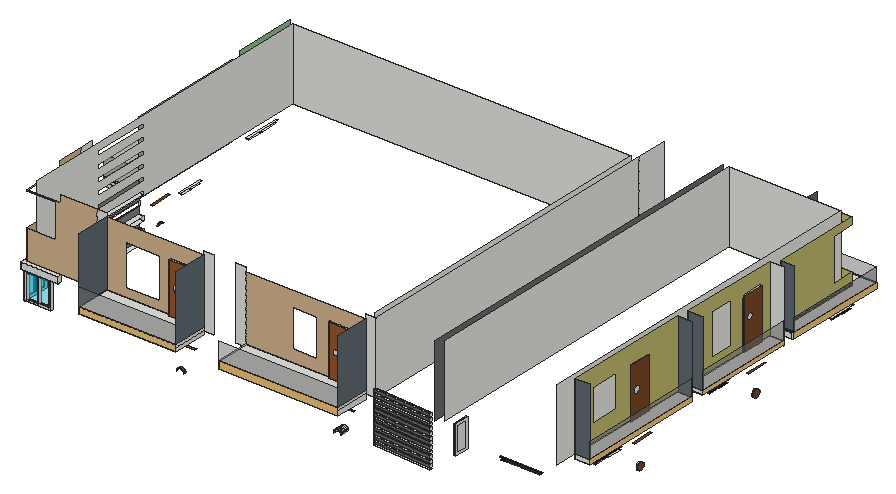
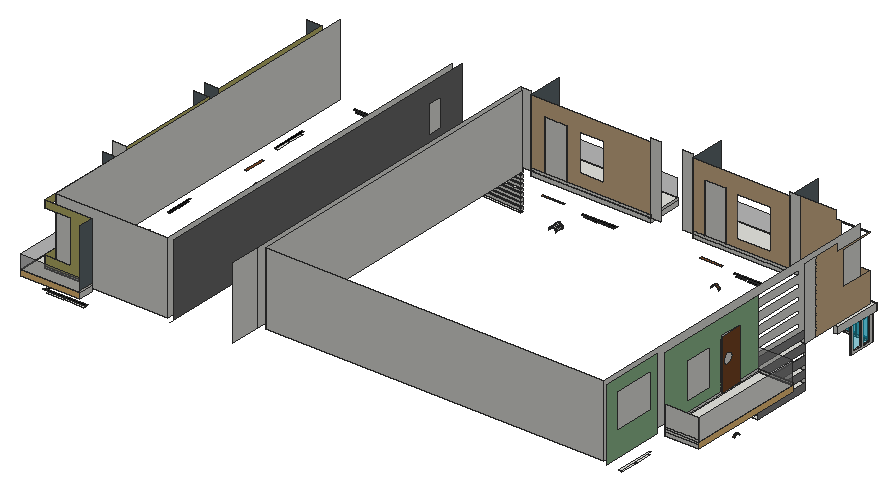
# SketchUp Ruby script. Lengths in inches.
U = 1.inch
M = Sketchup.active_model
def pt(a) = Geom::Point3d.new(a.map { |v| v * U })
def face(e, loops, mat)
  f = e.add_face(loops[0].map { |a| pt(a) })
  loops[1..].each { |l| e.add_face(l.map { |a| pt(a) }).erase! }
  f.material = f.back_material = mat if mat
  f
end
# faces: each face lists its corners as indices into pts; further lists are holes
def faces(e, pts, list, mat = nil) = list.each { |f| face(e, (f[0].is_a?(Array) ? f : [f]).map { |l| l.map { |i| pts[i] } }, mat) }
# xy, xz, yz: faces in a plane at the given z, y or x. An outline is a flat list of corners, or four numbers for a rectangle; further outlines are holes
def ring(l) = l.size == 4 ? [[l[0], l[1]], [l[2], l[1]], [l[2], l[3]], [l[0], l[3]]] : l.each_slice(2).to_a
def flat(e, list, mat, &to3) = list.each { |f| face(e, (f[0].is_a?(Array) ? f : [f]).map { |l| ring(l).map { |u, v| to3.(u, v) } }, mat) }
def xy(e, z, list, mat = nil) = flat(e, list, mat) { |x, y| [x, y, z] }
def xz(e, y, list, mat = nil) = flat(e, list, mat) { |x, z| [x, y, z] }
def yz(e, x, list, mat = nil) = flat(e, list, mat) { |y, z| [x, y, z] }
def lines(e, pts, list) = list.each { |a, b| e.add_line(pt(pts[a]), pt(pts[b])) }
# prism: a flat outline (further loops are holes) pulled along v
def prism(e, loops, v, mat = nil)
  f = face(e, loops, mat); d = Geom::Vector3d.new(v.map { |x| x * U })
  f.pushpull(f.normal.samedirection?(d) ? d.length : -d.length)
end
def box(e, o, s, mat = nil) = prism(e, [[o, [o[0] + s[0], o[1], o[2]], [o[0] + s[0], o[1] + s[1], o[2]], [o[0], o[1] + s[1], o[2]]]], [0, 0, s[2]], mat)
def at(x, y, z, deg = 0) = Geom::Transformation.translation(pt([x, y, z])) * Geom::Transformation.rotation(ORIGIN, Z_AXIS, deg.degrees)
def axes(o, x, y, z) = Geom::Transformation.new([*x, 0, *y, 0, *z, 0, *pt(o).to_a, 1])
def part(name) = M.definitions.add(name)
# library, detail: a bought-in or finely detailed component or shape, given as its bounding box
def library(name, o, s) = part(name).tap { |d| box(d.entities, o, s) }
def detail(e, o, s) = box(e.add_group.entities, o, s)
def put(e, d, t, mat = nil) = e.add_instance(d, t).tap { |i| i.material = mat if mat }
def group(e, t, mat = nil) = e.add_group.tap { |g| g.transformation = t; g.material = mat if mat }.entities
root = M.entities
M.materials.add("[0035_Tan]").color = [210, 180, 140]
M.materials.add("[0057_DarkKhaki]").color = [189, 183, 107]
M.materials.add("[0072_DarkSeaGreen]").color = [143, 188, 143]
M.materials.add("[0133_Gray]").color = [128, 128, 128]
M.materials.add("[0134_DimGray]").color = [105, 105, 105]
M.materials.add("[0137_Black]").color = [0, 0, 0]
M.materials.add("[Formica Speckled Grey]").color = [94, 105, 111]
M.materials.add("[Translucent Glass Gray]").color = [128, 128, 128]
M.materials["[Translucent Glass Gray]"].alpha = 0.5
M.materials.add("[Translucent Glass Tinted]").color = [8, 201, 241]
M.materials["[Translucent Glass Tinted]"].alpha = 0.48
M.materials.add("[Wood Cherry Original]").color = [152, 86, 42]
M.materials.add("[Wood OSB]").color = [240, 195, 122]
M.materials.add("[Wood Veneer 01]").color = [120, 70, 37]
xy(root,300.63,[[83.8125,295.24,92.8125,392.06]])
xy(root,300.91,[[763.41,201.89,766.41,227.45]])
xy(root,303.43,[[766.19,148.96,766.41,152.52,668.06,158.52,667.84,154.96]])
xy(root,303.91,[[763.41,204.89,766.41,224.45]])
xy(root,306.11,[[766.19,148.96,667.84,154.96,668.05,158.39,766.4,152.39],[766.4,152.39,668.05,158.39,668.06,158.52,766.41,152.52]])
xy(root,310.31,[[766.19,148.96,766.4,152.39,668.05,158.39,667.84,154.96],[766.4,152.39,766.41,152.52,668.06,158.52,668.05,158.39]])
xy(root,312.98,[[766.19,148.96,667.84,154.96,668.06,158.52,766.41,152.52]])
xy(root,313.12,[[83.8125,295.24,92.8125,392.06]])
xy(root,314.18,[[83.8125,155.58,126.6875,158.58]])
xy(root,314.24,[[80.8125,155.58,83.8125,155.71],[80.8125,155.71,83.8125,200.33]])
xy(root,317.18,[[766.19,148.96,766.41,152.52,668.06,158.52,667.84,154.96],[86.8125,155.58,105.25,158.58],[106.83,155.58,123.6875,158.58]])
xy(root,317.24,[[80.8125,161.58,83.8125,177.8],[80.8125,179.46,83.8125,197.33]])
xy(root,319.86,[[766.19,148.96,667.84,154.96,668.06,158.52,766.41,152.52]])
xy(root,320.56,[[83.8125,295.24,92.8125,392.06]])
xy(root,324.06,[[766.19,148.96,766.41,152.52,668.06,158.52,667.84,154.96]])
xy(root,326.73,[[766.19,148.96,667.84,154.96,668.06,158.52,766.41,152.52]])
xy(root,329.54,[[80.8125,483.71,83.8125,500.7],[80.8125,502.52,83.8125,521.33]])
xy(root,330.93,[[766.19,148.96,766.41,152.52,668.06,158.52,667.84,154.96]])
xy(root,332.54,[[80.8125,480.71,83.8125,524.33]])
xy(root,333.06,[[83.8125,295.24,92.8125,392.06]])
xy(root,333.34,[[267.42,155.58,288.08,158.58],[291.62,155.58,308.74,158.58]],"[0137_Black]")
xy(root,333.43,[[511.66,155.58,537.16,158.58],[540.07,155.58,562.66,158.58]],"[0137_Black]")
xy(root,333.61,[[766.19,148.96,667.84,154.96,668.06,158.52,766.41,152.52]])
xy(root,336.34,[[264.42,155.58,311.74,158.58]],"[0137_Black]")
xy(root,336.43,[[508.66,155.58,565.66,158.58]],"[0137_Black]")
xy(root,337.81,[[766.19,148.96,766.41,152.52,668.06,158.52,667.84,154.96]])
xy(root,340.06,[[80.8125,421.71,83.8125,457.71]],"[Wood Veneer 01]")
xy(root,340.47,[[332.04,155.58,368.04,158.58]],"[Wood Cherry Original]")
xy(root,340.48,[[766.19,148.96,667.84,154.96,668.06,158.52,766.41,152.52]])
xy(root,340.5,[[83.8125,295.24,92.8125,392.06]])
xy(root,340.72,[[596.81,155.58,632.81,158.58]],"[Wood Cherry Original]")
xy(root,343.18,[[972.47,553.32,975.47,589.32]],"[Wood Veneer 01]")
xy(root,343.44,[[972.47,315.42,975.47,351.42]],"[Wood Veneer 01]")
xy(root,344.68,[[766.19,148.96,766.41,152.52,668.06,158.52,667.84,154.96]])
xy(root,345.53,[[763.41,204.89,766.41,224.45]])
xy(root,346.83,[[972.47,234.45,975.47,260.01],[972.47,262.22,975.47,285.58]])
xy(root,347.28,[[906.22,770.48,937.84,773.48],[940.13,770.48,969.47,773.48]])
xy(root,347.28,[[972.47,728.48,975.47,747.98],[972.47,750.32,975.47,767.48]],"[0137_Black]")
xy(root,347.36,[[766.19,148.96,667.84,154.96,668.06,158.52,766.41,152.52]])
xy(root,348.53,[[763.41,201.89,766.41,227.45]])
xy(root,349.41,[[972.47,471.54,975.47,490.38],[972.47,492.52,975.47,509.23]],"[0137_Black]")
xy(root,349.83,[[972.47,231.45,975.47,288.58]],"[0137_Black]")
xy(root,350.04,[[80.8125,623.08,83.8125,648.35],[80.8125,651.58,83.8125,680.08]])
xy(root,350.28,[[972.47,725.48,975.47,770.48]])
xy(root,350.28,[[903.22,770.48,972.47,773.48],[972.47,770.48,975.47,773.48]],"[0137_Black]")
xy(root,351.56,[[766.19,148.96,766.41,152.52,668.06,158.52,667.84,154.96]])
xy(root,352.41,[[972.47,468.54,975.47,512.23]],"[0137_Black]")
xy(root,353,[[83.8125,295.24,85.75,392.06]])
xy(root,353.04,[[80.8125,620.08,83.8125,683.08]])
xy(root,354.23,[[766.19,148.96,667.84,154.96,668.06,158.52,766.41,152.52]])
xy(root,355.59,[[914.48,155.58,916.69,158.58]])
xy(root,355.59,[[880.02,155.58,912.27,158.58],[912.27,155.58,914.48,158.58],[916.69,155.58,944.52,158.58]],"[0137_Black]")
xy(root,357.74,[[86.8125,155.58,105.25,158.58],[106.83,155.58,123.6875,158.58],[80.8125,161.58,83.8125,177.8],[80.8125,179.46,83.8125,197.33]])
xy(root,358.43,[[766.19,148.96,766.41,152.52,668.06,158.52,667.84,154.96]])
xy(root,358.59,[[877.02,155.58,947.52,158.58]],"[0137_Black]")
xy(root,360.44,[[83.8125,295.24,85.75,392.06]])
xy(root,360.74,[[77.8125,152.58,77.8125,232.98,83.8125,232.98,83.8125,200.33,80.8125,200.33,80.8125,155.58,126.6875,155.58,126.6875,158.58,141.375,158.58,141.375,152.58],[80.8125,155.58,83.8125,155.71],[83.8125,155.58,126.6875,158.58],[80.8125,155.71,83.8125,200.33]])
xy(root,361.48,[[766.19,148.96,667.84,154.96,668.06,158.52,766.41,152.52]])
xy(root,362.62,[[26.03,392.06,83.8125,587.65]],"[Wood OSB]")
xy(root,364.37,[[450.92,100.8,651.23,158.58]],"[Wood OSB]")
xy(root,365.68,[[766.19,148.96,766.41,152.52,668.06,158.52,667.84,154.96]])
xy(root,366.18,[[217.79,100.8,379.72,158.58]],"[Wood OSB]")
xy(root,368.73,[[766.19,148.96,667.84,154.96,668.06,158.52,766.41,152.52]])
xy(root,372.18,[[77.8125,152.58,141.375,152.58,141.375,158.58,83.8125,158.58,83.8125,232.98,77.8125,232.98],[26.03,392.06,83.8125,587.65]])
xy(root,372.18,[[972.47,194.93,996.47,408.53]],"[Wood OSB]")
xy(root,372.33,[[975.47,621.6875,975.47,770.48,896.3125,770.48,896.3125,794.48,996.47,794.48,996.47,621.6875]],"[Wood OSB]")
xy(root,372.5,[[972.47,431.23,996.47,600.85]],"[Wood OSB]")
xy(root,372.93,[[766.19,148.96,766.41,152.52,668.06,158.52,667.84,154.96],[83.8125,295.24,92.8125,392.06]])
xy(root,375.98,[[766.19,148.96,667.84,154.96,668.06,158.52,766.41,152.52]])
xy(root,376.06,[[80.8125,433.46,83.8125,469.46]])
xy(root,376.47,[[217.79,100.8,379.72,100.8,379.72,158.58,360.41,158.58,360.41,155.58,324.41,155.58,324.41,158.58,217.79,158.58],[324.41,155.58,360.41,158.58]])
xy(root,376.6,[[450.92,100.8,651.23,100.8,651.23,158.58,627.01,158.58,627.01,155.58,591.01,155.58,591.01,158.58,450.92,158.58],[591.01,155.58,627.01,158.58]])
xy(root,378.87,[[972.47,431.23,996.47,431.23,996.47,600.85,972.47,600.85,972.47,581.86,975.47,581.86,975.47,545.86,972.47,545.86],[972.47,545.86,975.47,581.86]])
xy(root,379.19,[[972.47,194.93,996.47,194.93,996.47,408.53,972.47,408.53,972.47,344.12,975.47,344.12,975.47,308.12,972.47,308.12],[972.47,308.12,975.47,344.12]])
xy(root,380.18,[[766.19,148.96,766.41,152.52,668.06,158.52,667.84,154.96]])
xy(root,380.38,[[83.8125,295.24,92.8125,392.06]])
xy(root,381.33,[[975.47,621.6875,996.47,621.6875,996.47,794.48,896.3125,794.48,896.3125,770.48,975.47,770.48]])
xy(root,383.23,[[766.19,148.96,667.84,154.96,668.06,158.52,766.41,152.52]])
xy(root,387.43,[[766.19,148.96,766.41,152.52,668.06,158.52,667.84,154.96]])
xz(root,100.8,[[217.79,376.47,379.72,406.08],[450.92,376.6,651.23,406.95]],"[Translucent Glass Gray]")
xz(root,100.8,[[450.92,364.37,651.23,376.6],[217.79,366.18,379.72,376.47]],"[Wood OSB]")
xz(root,152.58,[[77.8125,360.74,141.375,372.18]])
xz(root,155.58,[[[83.8125,314.18,126.6875,314.18,126.6875,360.74,80.8125,360.74,80.8125,314.24,83.8125,314.24],[86.8125,317.18,105.25,357.74],[106.83,317.18,123.6875,357.74]]])
xz(root,155.58,[[[324.41,376.47,360.41,460.47],[337.43,413.47,335.75,413.69,334.18,414.34,332.84,415.375,331.8,416.72,331.15,418.29,330.93,419.97,331.15,421.65,331.8,423.22,332.84,424.57,334.18,425.6,335.75,426.25,337.43,426.47,339.12,426.25,340.68,425.6,342.03,424.57,343.0625,423.22,343.71,421.65,343.93,419.97,343.71,418.29,343.0625,416.72,342.03,415.375,340.68,414.34,339.12,413.69]],[[591.01,376.6,627.01,460.6],[603.27,413.39,601.96,413.5625,600.74,414.07,599.69,414.87,598.89,415.92,598.38,417.14,598.21,418.45,598.38,419.76,598.89,420.98,599.69,422.03,600.74,422.83,601.96,423.34,603.27,423.51,604.58,423.34,605.81,422.83,606.85,422.03,607.66,420.98,608.16,419.76,608.34,418.45,608.16,417.14,607.66,415.92,606.85,414.87,605.81,414.07,604.58,413.5625]]],"[Wood Cherry Original]")
xz(root,158.58,[[[83.8125,314.18,126.6875,360.74],[86.8125,317.18,105.25,357.74],[106.83,317.18,123.6875,357.74]],[450.92,364.37,651.23,372.18],[217.79,366.18,379.72,372.18],[200.97,372.18,217.79,492.18],[217.79,372.18,379.72,376.47],
  [379.72,372.18,396.54,492.18],[434.03,372.18,450.85,492.18],[450.92,372.18,651.23,372.31],[651.23,372.18,668.06,492.18],[765.79,372.18,766.41,492.18],
  [450.92,372.31,651.23,376.6],[324.41,376.47,360.41,460.47],[591.01,376.6,627.01,460.6]])
xz(root,158.58,[[83.8125,372.18,200.97,372.18,200.97,492.18,140.48,492.18,140.48,479.56,83.8125,479.56,83.8125,477.85,132.6875,477.85,132.6875,421.66,83.8125,421.66],[[450.85,372.18,450.92,372.18,450.92,376.6,591.01,376.6,591.01,460.6,627.01,460.6,627.01,376.6,651.23,376.6,651.23,485.43,450.92,485.43,450.92,492.18,450.85,492.18],[528.12,396.63,569.87,459.19]],[[217.79,376.47,324.41,376.47,324.41,460.47,360.41,460.47,360.41,376.47,379.72,376.47,379.72,486.18,217.79,486.18],[249.03,390.84,306.03,458.71]]],"[0035_Tan]")
xz(root,158.58,[[86.8125,317.18,105.25,357.74],[106.83,317.18,123.6875,357.74]],"[Translucent Glass Tinted]")
xz(root,161.58,[[80.8125,317.24,83.8125,357.74]])
xz(root,177.8,[[80.8125,317.24,83.8125,357.74]])
xz(root,179.46,[[80.8125,317.24,83.8125,357.74]])
xz(root,194.93,[[972.47,372.18,996.47,379.19]])
xz(root,194.93,[[972.47,379.19,996.47,492.18]],"[Formica Speckled Grey]")
xz(root,197.33,[[80.8125,317.24,83.8125,357.74]])
xz(root,200.33,[[80.8125,314.24,83.8125,360.74]])
xz(root,201.89,[[763.41,300.91,766.41,348.53]])
xz(root,204.89,[[763.41,303.91,766.41,345.53]])
xz(root,224.45,[[763.41,303.91,766.41,345.53]])
xz(root,227.45,[[763.41,300.91,766.41,348.53]])
xz(root,232.98,[[77.8125,360.74,83.8125,372.18]])
xz(root,295.24,[[83.8125,313.12,92.8125,320.56],[83.8125,333.06,92.8125,340.5],[83.8125,353,85.75,360.44],[83.8125,372.93,92.8125,380.38]])
xz(root,308.12,[[972.47,379.19,975.47,463.19]],"[Wood Veneer 01]")
xz(root,344.12,[[972.47,379.19,975.47,463.19]],"[Wood Veneer 01]")
xz(root,392.06,[[83.8125,313.12,92.8125,320.56],[83.8125,333.06,92.8125,340.5],[83.8125,353,85.75,360.44],[26.03,362.62,83.8125,368.62],[26.03,368.62,83.8125,372.18],
  [26.03,372.18,83.8125,372.56],[26.03,372.56,83.8125,372.93],[26.03,372.93,83.8125,376.06],[83.8125,372.93,92.8125,380.38]])
xz(root,392.06,[[26.03,376.06,83.8125,409.83]],"[Translucent Glass Gray]")
xz(root,408.53,[[972.47,372.18,996.47,379.19]])
xz(root,408.53,[[972.47,379.19,996.47,492.18]],"[Formica Speckled Grey]")
xz(root,431.23,[[972.47,372.18,996.47,372.5],[972.47,372.5,996.47,378.87]])
xz(root,431.23,[[972.47,378.87,996.47,489.56]],"[Formica Speckled Grey]")
xz(root,433.46,[[80.8125,376.06,83.8125,460.06]],"[Wood Veneer 01]")
xz(root,469.46,[[80.8125,376.06,83.8125,460.06]],"[Wood Veneer 01]")
xz(root,545.86,[[972.47,378.87,975.47,462.87]],"[Wood Veneer 01]")
xz(root,581.86,[[972.47,378.87,975.47,462.87]],"[Wood Veneer 01]")
xz(root,587.65,[[26.03,362.62,83.8125,368.62],[26.03,368.62,83.8125,372.18],[26.03,372.18,83.8125,376.06],[26.03,376.06,83.8125,409.42]])
xz(root,600.85,[[972.47,372.18,996.47,372.5],[972.47,372.5,996.47,378.87],[972.47,378.87,996.47,489.56]])
xz(root,621.6875,[[975.47,372.33,993.47,381.33],[993.47,372.33,996.47,381.33],[975.47,381.33,993.47,381.52],[993.47,381.33,996.47,381.52],[975.47,381.52,993.47,383.71],
  [993.47,381.52,996.47,383.71],[975.47,383.71,993.47,384.33],[993.47,383.71,996.47,384.33]])
xz(root,621.6875,[[975.47,384.33,996.47,482.83]],"[Formica Speckled Grey]")
xz(root,703.7,[[92.8125,372.18,659.06,492.18]])
xz(root,761.48,[[775.41,372.18,963.47,492.18]])
xz(root,770.48,[[896.3125,372.33,918.4,381.33],[918.4,372.33,975.47,381.33],[896.3125,381.33,918.4,384.33],[918.4,381.33,975.47,384.33]])
xz(root,770.48,[[896.3125,384.33,896.3125,482.83,975.47,482.83,975.47,471.13,931.65,471.13,931.65,400.19,975.47,400.19,975.47,384.33]],"[0057_DarkKhaki]")
xz(root,794.48,[[896.3125,381.33,996.47,405.05]],"[Translucent Glass Gray]")
xz(root,794.48,[[896.3125,372.33,996.47,381.33]],"[Wood OSB]")
yz(root,26.03,[[392.06,372.18,587.65,409.42]],"[Translucent Glass Gray]")
yz(root,26.03,[[392.06,362.62,587.65,372.18]],"[Wood OSB]")
yz(root,77.8125,[[152.58,360.74,232.98,372.18]])
yz(root,80.8125,[[155.58,314.24,155.71,360.74],[[155.71,314.24,200.33,360.74],[179.46,317.24,197.33,357.74],[161.58,317.24,177.8,357.74]]])
yz(root,80.8125,[[[433.46,376.06,469.46,460.06],[458.74,414.24,461.07,414.54,463.24,415.44,465.1,416.87,466.53,418.74,467.43,420.91,467.74,423.24,467.43,425.57,466.53,427.74,465.1,429.6,463.24,431.03,461.07,431.93,458.74,432.24,456.41,431.93,454.24,431.03,452.375,429.6,450.95,427.74,450.05,425.57,449.74,423.24,450.05,420.91,450.95,418.74,452.375,416.87,454.24,415.44,456.41,414.54]]],"[Wood Veneer 01]")
yz(root,83.8125,[[155.58,314.18,158.58,314.24],[[158.58,314.24,200.33,360.74],[179.46,317.24,197.33,357.74],[161.58,317.24,177.8,357.74]],[392.06,362.62,587.65,368.62],[392.06,368.62,587.65,372.18],[271.7,372.18,295.24,492.18],
  [392.06,372.18,587.65,376.06],[433.46,376.06,469.46,460.06]])
yz(root,83.8125,[[158.58,372.18,158.58,421.47,214.96,421.47,214.96,477.85,158.58,477.85,158.58,479.56,227.52,479.56,227.52,492.18,271.7,492.18,271.7,372.18]],"[0035_Tan]")
yz(root,83.8125,[[[604.3125,372.18,709.05,492.18],[615.71,412.82,687.27,471.63]],[[392.06,376.06,392.06,486.18,587.65,486.18,587.65,376.06,469.46,376.06,469.46,460.06,433.46,460.06,433.46,376.06],[493.7,392.41,541.45,453.73]]],"[0072_DarkSeaGreen]")
yz(root,83.8125,[[295.24,300.63,392.06,313.12],[295.24,320.56,392.06,333.06],[295.24,340.5,392.06,353],[295.24,360.44,392.06,372.93],[295.24,380.38,392.06,392.87]],"[0133_Gray]")
yz(root,83.8125,[[161.58,317.24,177.8,357.74],[179.46,317.24,197.33,357.74]],"[Translucent Glass Tinted]")
yz(root,86.8125,[[155.58,317.18,158.58,357.74]])
yz(root,92.8125,[[[167.58,372.18,703.7,492.18],[295.24,472.62,392.06,480.06],[295.24,452.68,392.06,460.13],[295.24,432.75,392.06,440.19],[295.24,412.81,392.06,420.25],[295.24,392.87,392.06,400.31],[295.24,372.93,392.06,380.38]]])
yz(root,105.25,[[155.58,317.18,158.58,357.74]])
yz(root,106.83,[[155.58,317.18,158.58,357.74]])
yz(root,123.6875,[[155.58,317.18,158.58,357.74]])
yz(root,126.6875,[[155.58,314.18,158.58,360.74]])
yz(root,141.375,[[152.58,360.74,158.58,360.87],[152.58,360.87,158.58,372.18]])
yz(root,217.79,[[100.8,366.18,158.58,372.18],[100.8,372.18,158.58,376.47]])
yz(root,217.79,[[100.8,376.47,158.58,486.18]],"[Formica Speckled Grey]")
yz(root,324.41,[[155.58,376.47,158.58,460.47]],"[Wood Cherry Original]")
yz(root,360.41,[[155.58,376.47,158.58,460.47]],"[Wood Cherry Original]")
yz(root,379.72,[[100.8,366.18,158.58,372.18],[100.8,372.18,158.58,376.47]])
yz(root,379.72,[[100.8,376.47,158.58,486.18]],"[Formica Speckled Grey]")
yz(root,450.92,[[100.8,364.37,158.58,372.31],[100.8,372.31,158.58,376.6]])
yz(root,591.01,[[155.58,376.6,158.58,460.6]],"[Wood Cherry Original]")
yz(root,627.01,[[155.58,376.6,158.58,460.6]],"[Wood Cherry Original]")
yz(root,651.23,[[100.8,364.37,158.58,372.31],[100.8,372.31,158.58,376.6]])
yz(root,651.23,[[100.8,376.6,158.58,485.43]],"[Formica Speckled Grey]")
yz(root,659.06,[[167.58,372.18,703.7,492.18]])
yz(root,668.06,[[158.58,372.18,709.05,492.18],[709.05,372.18,761.48,492.18]])
yz(root,763.41,[[[201.89,300.91,227.45,348.53],[204.89,303.91,224.45,345.53]]])
yz(root,766.41,[[[201.89,300.91,227.45,348.53],[204.89,303.91,224.45,345.53]],[204.89,303.91,224.45,345.53]])
yz(root,766.41,[[[158.58,372.18,761.48,492.18],[201.89,414.22,227.45,461.85]]],"[0134_DimGray]")
yz(root,775.41,[[167.58,372.18,761.48,492.18]])
yz(root,896.3125,[[770.48,372.33,794.48,381.33],[770.48,381.33,794.48,384.33]])
yz(root,896.3125,[[770.48,384.33,794.48,482.83]],"[Formica Speckled Grey]")
yz(root,963.47,[[167.58,372.18,761.48,492.18]])
yz(root,972.47,[[194.93,372.18,408.53,379.19],[431.23,372.18,600.85,372.5],[431.23,372.5,600.85,378.87],[545.86,378.87,581.86,462.87],[308.12,379.19,344.12,463.19]])
yz(root,972.47,[[[431.23,378.87,545.86,378.87,545.86,462.87,581.86,462.87,581.86,378.87,600.85,378.87,600.85,489.56,431.23,489.56],[480.96,397.87,521.21,466.75]],[[194.93,379.19,308.12,379.19,308.12,463.19,344.12,463.19,344.12,379.19,408.53,379.19,408.53,492.18,194.93,492.18],[230.61,409.32,280.48,463.01]]],"[0057_DarkKhaki]")
yz(root,975.47,[[324.66,300.15,323.16,300.35,321.76,300.93,320.55,301.85,319.63,303.05,319.05,304.46,318.85,305.96,319.05,307.46,319.63,308.87,320.55,310.07,321.76,310.99,323.16,311.57,324.66,311.77,326.17,311.57,327.57,310.99,328.77,310.07,329.7,308.87,330.28,307.46,330.47,305.96,330.28,304.46,329.7,303.05,328.77,301.85,327.57,300.93,326.17,300.35],[566.66,302.99,565.11,303.19,563.66,303.79,562.42,304.75,561.46,305.99,560.86,307.4375,560.66,308.99,560.86,310.54,561.46,311.99,562.42,313.23,563.66,314.19,565.11,314.78,566.66,314.99,568.21,314.78,569.66,314.19,570.9,313.23,571.86,311.99,572.46,310.54,572.66,308.99,572.46,307.4375,571.86,305.99,570.9,304.75,569.66,303.79,568.21,303.19],[621.6875,372.33,770.48,381.33],[621.6875,381.33,770.48,381.52],[621.6875,381.52,770.48,383.71],
  [621.6875,383.71,770.48,384.33]])
yz(root,975.47,[[621.6875,384.33,770.48,384.33,770.48,400.19,731.11,400.19,731.11,471.13,770.48,471.13,770.48,482.83,621.6875,482.83]],"[0057_DarkKhaki]")
yz(root,975.47,[[[545.86,378.87,581.86,462.87],[556.25,422.52,554.76,422.71,553.38,423.29,552.1875,424.2,551.27,425.39,550.7,426.78,550.5,428.27,550.7,429.76,551.27,431.14,552.1875,432.33,553.38,433.25,554.76,433.82,556.25,434.02,557.74,433.82,559.13,433.25,560.32,432.33,561.23,431.14,561.81,429.76,562,428.27,561.81,426.78,561.23,425.39,560.32,424.2,559.13,423.29,557.74,422.71]],[[308.12,379.19,344.12,463.19],[319.91,416.2,318.33,416.41,316.85,417.02,315.58,418,314.61,419.26,314,420.74,313.79,422.33,314,423.91,314.61,425.39,315.58,426.66,316.85,427.63,318.33,428.24,319.91,428.45,321.5,428.24,322.98,427.63,324.25,426.66,325.22,425.39,325.83,423.91,326.04,422.33,325.83,420.74,325.22,419.26,324.25,418,322.98,417.02,321.5,416.41]]],"[Wood Veneer 01]")
yz(root,978.47,[[324.66,300.15,326.17,300.35,327.57,300.93,328.77,301.85,329.7,303.05,330.28,304.46,330.47,305.96,330.28,307.46,329.7,308.87,328.77,310.07,327.57,310.99,326.17,311.57,324.66,311.77,323.16,311.57,321.76,310.99,320.55,310.07,319.63,308.87,319.05,307.46,318.85,305.96,319.05,304.46,319.63,303.05,320.55,301.85,321.76,300.93,323.16,300.35],[566.66,302.99,568.21,303.19,569.66,303.79,570.9,304.75,571.86,305.99,572.46,307.4375,572.66,308.99,572.46,310.54,571.86,311.99,570.9,313.23,569.66,314.19,568.21,314.78,566.66,314.99,565.11,314.78,563.66,314.19,562.42,313.23,561.46,311.99,560.86,310.54,560.66,308.99,560.86,307.4375,561.46,305.99,562.42,304.75,563.66,303.79,565.11,303.19]],"[Wood Veneer 01]")
yz(root,996.47,[[431.23,378.87,600.85,409.09],[194.93,379.19,408.53,406.57],[621.6875,381.33,794.48,405.05]],"[Translucent Glass Gray]")
yz(root,996.47,[[194.93,372.18,408.53,379.19],[621.6875,372.33,794.48,381.33],[431.23,372.5,600.85,378.87]],"[Wood OSB]")
p = [[602.35,155.58,301.37],[602.54,155.58,299.88],[602.54,152.58,299.88],[602.35,152.58,301.37],[613.65,155.58,299.88],[613.85,155.58,301.37],
  [613.85,152.58,301.37],[613.65,152.58,299.88],[602.35,167.52,301.37],[602.54,167.52,299.88],[613.65,167.52,299.88],[613.85,167.52,301.37],
  [339.32,155.58,301.73],[339.1,155.58,300.08],[339.1,152.58,300.08],[339.32,152.58,301.73],[351.85,155.58,300.08],[351.64,155.58,301.73],
  [351.64,152.58,301.73],[351.85,152.58,300.08],[975.47,323.16,300.35],[975.47,324.66,300.15],[978.47,324.66,300.15],[978.47,323.16,300.35],
  [975.47,326.17,300.35],[978.47,326.17,300.35],[975.47,321.76,300.93],[978.47,321.76,300.93],[975.47,327.57,300.93],[978.47,327.57,300.93],
  [80.8125,438.43,300.73],[80.8125,439.35,301.93],[77.8125,439.35,301.93],[77.8125,438.43,300.73],[80.8125,447.48,301.93],[80.8125,448.39,300.73],
  [77.8125,448.39,300.73],[77.8125,447.48,301.93],[975.47,320.55,301.85],[978.47,320.55,301.85],[975.47,328.77,301.85],[978.47,328.77,301.85],
  [602.54,155.58,302.85],[602.54,152.58,302.85],[613.65,155.58,302.85],[613.65,152.58,302.85],[602.54,167.52,302.85],[613.65,167.52,302.85],
  [339.96,155.58,303.27],[339.96,152.58,303.27],[351,155.58,303.27],[351,152.58,303.27],[975.47,319.63,303.05],[978.47,319.63,303.05],
  [975.47,329.7,303.05],[978.47,329.7,303.05],[80.8125,440.54,302.84],[77.8125,440.54,302.84],[80.8125,446.29,302.84],[77.8125,446.29,302.84],
  [80.8125,441.92,303.41],[77.8125,441.92,303.41],[80.8125,444.9,303.41],[77.8125,444.9,303.41],[603.12,155.58,304.24],[603.12,152.58,304.24],
  [613.08,155.58,304.24],[613.08,152.58,304.24],[603.12,167.52,304.24],[613.08,167.52,304.24],[975.47,565.11,303.19],[975.47,566.66,302.99],
  [978.47,566.66,302.99],[978.47,565.11,303.19],[975.47,568.21,303.19],[978.47,568.21,303.19],[975.47,319.05,304.46],[978.47,319.05,304.46],
  [975.47,330.28,304.46],[978.47,330.28,304.46],[975.47,563.66,303.79],[978.47,563.66,303.79],[975.47,569.66,303.79],[978.47,569.66,303.79],
  [340.97,155.58,304.59],[340.97,152.58,304.59],[349.99,155.58,304.59],[349.99,152.58,304.59],[80.8125,443.41,303.61],[77.8125,443.41,303.61],
  [975.47,562.42,304.75],[978.47,562.42,304.75],[975.47,570.9,304.75],[978.47,570.9,304.75],[604.03,155.58,305.43],[604.03,152.58,305.43],
  [612.16,155.58,305.43],[612.16,152.58,305.43],[604.03,167.52,305.43],[612.16,167.52,305.43],[975.47,318.85,305.96],[978.47,318.85,305.96],
  [975.47,330.47,305.96],[978.47,330.47,305.96],[342.29,155.58,305.6],[342.29,152.58,305.6],[348.67,155.58,305.6],[348.67,152.58,305.6],
  [975.47,561.46,305.99],[978.47,561.46,305.99],[975.47,571.86,305.99],[978.47,571.86,305.99],[605.22,155.58,306.35],[605.22,152.58,306.35],
  [610.97,155.58,306.35],[610.97,152.58,306.35],[605.22,167.52,306.35],[610.97,167.52,306.35],[343.83,155.58,306.24],[343.83,152.58,306.24],
  [347.13,155.58,306.24],[347.13,152.58,306.24],[975.47,319.05,307.46],[978.47,319.05,307.46],[975.47,330.28,307.46],[978.47,330.28,307.46],
  [975.47,560.86,307.4375],[978.47,560.86,307.4375],[975.47,572.46,307.4375],[978.47,572.46,307.4375],[766.19,148.96,310.31],[667.84,154.96,310.31],
  [667.84,154.96,306.11],[766.19,148.96,306.11],[766.4,152.39,306.11],[766.4,152.39,310.31],[668.05,158.39,310.31],[668.05,158.39,306.11],
  [766.41,152.52,306.11],[766.41,152.52,310.31],[668.06,158.52,310.31],[668.06,158.52,306.11],[345.48,155.58,306.46],[345.48,152.58,306.46],
  [606.61,155.58,306.92],[606.61,152.58,306.92],[609.59,155.58,306.92],[609.59,152.58,306.92],[606.61,167.52,306.92],[609.59,167.52,306.92],
  [608.1,155.58,307.12],[608.1,152.58,307.12],[608.1,167.52,307.12],[975.47,560.66,308.99],[978.47,560.66,308.99],[975.47,572.66,308.99],
  [978.47,572.66,308.99],[975.47,319.63,308.87],[978.47,319.63,308.87],[975.47,329.7,308.87],[978.47,329.7,308.87],[975.47,320.55,310.07],
  [978.47,320.55,310.07],[975.47,328.77,310.07],[978.47,328.77,310.07],[975.47,560.86,310.54],[978.47,560.86,310.54],[975.47,572.46,310.54],
  [978.47,572.46,310.54],[975.47,321.76,310.99],[978.47,321.76,310.99],[975.47,327.57,310.99],[978.47,327.57,310.99],[975.47,561.46,311.99],
  [978.47,561.46,311.99],[975.47,571.86,311.99],[978.47,571.86,311.99],[975.47,323.16,311.57],[978.47,323.16,311.57],[975.47,326.17,311.57],
  [978.47,326.17,311.57],[975.47,324.66,311.77],[978.47,324.66,311.77],[975.47,562.42,313.23],[978.47,562.42,313.23],[975.47,570.9,313.23],
  [978.47,570.9,313.23],[766.19,148.96,317.18],[667.84,154.96,317.18],[667.84,154.96,312.98],[766.19,148.96,312.98],[766.41,152.52,312.98],
  [766.41,152.52,317.18],[668.06,158.52,317.18],[668.06,158.52,312.98],[975.47,563.66,314.19],[978.47,563.66,314.19],[975.47,569.66,314.19],
  [978.47,569.66,314.19],[975.47,565.11,314.78],[978.47,565.11,314.78],[975.47,568.21,314.78],[978.47,568.21,314.78],[975.47,566.66,314.99],
  [978.47,566.66,314.99],[766.19,148.96,324.06],[667.84,154.96,324.06],[667.84,154.96,319.86],[766.19,148.96,319.86],[766.41,152.52,319.86],
  [766.41,152.52,324.06],[668.06,158.52,324.06],[668.06,158.52,319.86],[766.19,148.96,330.93],[667.84,154.96,330.93],[667.84,154.96,326.73],
  [766.19,148.96,326.73],[766.41,152.52,326.73],[766.41,152.52,330.93],[668.06,158.52,330.93],[668.06,158.52,326.73],[766.19,148.96,337.81],
  [667.84,154.96,337.81],[667.84,154.96,333.61],[766.19,148.96,333.61],[766.41,152.52,333.61],[766.41,152.52,337.81],[668.06,158.52,337.81],
  [668.06,158.52,333.61],[766.19,148.96,344.68],[667.84,154.96,344.68],[667.84,154.96,340.48],[766.19,148.96,340.48],[766.41,152.52,340.48],
  [766.41,152.52,344.68],[668.06,158.52,344.68],[668.06,158.52,340.48],[766.19,148.96,351.56],[667.84,154.96,351.56],[667.84,154.96,347.36],
  [766.19,148.96,347.36],[766.41,152.52,347.36],[766.41,152.52,351.56],[668.06,158.52,351.56],[668.06,158.52,347.36],[766.19,148.96,358.43],
  [667.84,154.96,358.43],[667.84,154.96,354.23],[766.19,148.96,354.23],[766.41,152.52,354.23],[766.41,152.52,358.43],[668.06,158.52,358.43],
  [668.06,158.52,354.23],[766.19,148.96,365.68],[667.84,154.96,365.68],[667.84,154.96,361.48],[766.19,148.96,361.48],[766.41,152.52,361.48],
  [766.41,152.52,365.68],[668.06,158.52,365.68],[668.06,158.52,361.48],[766.19,148.96,372.93],[667.84,154.96,372.93],[667.84,154.96,368.73],
  [766.19,148.96,368.73],[766.41,152.52,368.73],[766.41,152.52,372.93],[668.06,158.52,372.93],[668.06,158.52,368.73],[668.06,158.58,492.18],
  [668.06,158.58,372.18],[668.05,158.52,372.18],[668.05,158.52,492.18],[766.19,148.96,380.18],[667.84,154.96,380.18],[667.84,154.96,375.98],
  [766.19,148.96,375.98],[766.41,152.52,375.98],[766.41,152.52,380.18],[668.06,158.52,380.18],[668.06,158.52,375.98],[766.19,148.96,387.43],
  [667.84,154.96,387.43],[667.84,154.96,383.23],[766.19,148.96,383.23],[766.41,152.52,383.23],[766.41,152.52,387.43],[668.06,158.52,387.43],
  [668.06,158.52,383.23],[766.41,761.48,372.18],[766.41,770.48,372.18]]
faces(root,p,[[0,1,2,3],[4,5,6,7],[12,13,14,15],[16,17,18,19],[42,0,3,43],[5,44,45,6],[48,12,15,49],[17,50,51,18],
  [64,42,43,65],[44,66,67,45],[84,48,49,85],[50,86,87,51],[94,64,65,95],[66,96,97,67],[104,84,85,105],[86,106,107,87],
  [112,94,95,113],[96,114,115,97],[118,104,105,119],[106,120,121,107],[142,118,119,143],[120,142,143,121],[144,112,113,145],[114,146,147,115],
  [150,144,145,151],[146,150,151,147]],"[Wood Cherry Original]")
faces(root,p,[[1,0,8,9],[5,4,10,11],[0,42,46,8],[44,5,11,47],[42,64,68,46],[66,44,47,69],[64,94,98,68],[96,66,69,99],
  [94,112,116,98],[114,96,99,117],[134,135,130,133],[136,135,134,137],[138,139,135,134],[140,139,138,141],[136,137,132,131],[140,141,137,136],
  [112,144,148,116],[146,114,117,149],[144,150,152,148],[150,146,149,152],[191,192,187,190],[193,192,191,194],[193,194,189,188],[209,210,205,208],
  [211,210,209,212],[211,212,207,206],[217,218,213,216],[219,218,217,220],[219,220,215,214],[225,226,221,224],[227,226,225,228],[227,228,223,222],
  [233,234,229,232],[235,234,233,236],[235,236,231,230],[241,242,237,240],[243,242,241,244],[243,244,239,238],[249,250,245,248],[251,250,249,252],
  [251,252,247,246],[257,258,253,256],[259,258,257,260],[259,260,255,254],[265,266,261,264],[267,266,265,268],[267,268,263,262],[269,270,271,272],
  [277,278,273,276],[279,278,277,280],[279,280,275,274],[285,286,281,284],[287,286,285,288],[287,288,283,282]])
faces(root,p,[[20,21,22,23],[21,24,25,22],[26,20,23,27],[24,28,29,25],[30,31,32,33],[34,35,36,37],[38,26,27,39],[28,40,41,29],
  [52,38,39,53],[40,54,55,41],[31,56,57,32],[58,34,37,59],[56,60,61,57],[62,58,59,63],[70,71,72,73],[71,74,75,72],
  [76,52,53,77],[54,78,79,55],[80,70,73,81],[74,82,83,75],[60,88,89,61],[88,62,63,89],[90,80,81,91],[82,92,93,83],
  [100,76,77,101],[78,102,103,79],[108,90,91,109],[92,110,111,93],[122,100,101,123],[102,124,125,103],[126,108,109,127],[110,128,129,111],
  [153,126,127,154],[128,155,156,129],[157,122,123,158],[124,159,160,125],[161,157,158,162],[159,163,164,160],[165,153,154,166],[155,167,168,156],
  [169,161,162,170],[163,171,172,164],[173,165,166,174],[167,175,176,168],[177,169,170,178],[171,179,180,172],[181,177,178,182],[179,181,182,180],
  [183,173,174,184],[175,185,186,176],[195,183,184,196],[185,197,198,186],[199,195,196,200],[197,201,202,198],[203,199,200,204],[201,203,204,202]],"[Wood Veneer 01]")
faces(root,p,[[130,131,132,133],[187,188,189,190],[205,206,207,208],[213,214,215,216],[221,222,223,224],[229,230,231,232],[237,238,239,240],[245,246,247,248],
  [253,254,255,256],[261,262,263,264],[273,274,275,276],[281,282,283,284]],"[0134_DimGray]")
lines(root,p,[[289,290]])
